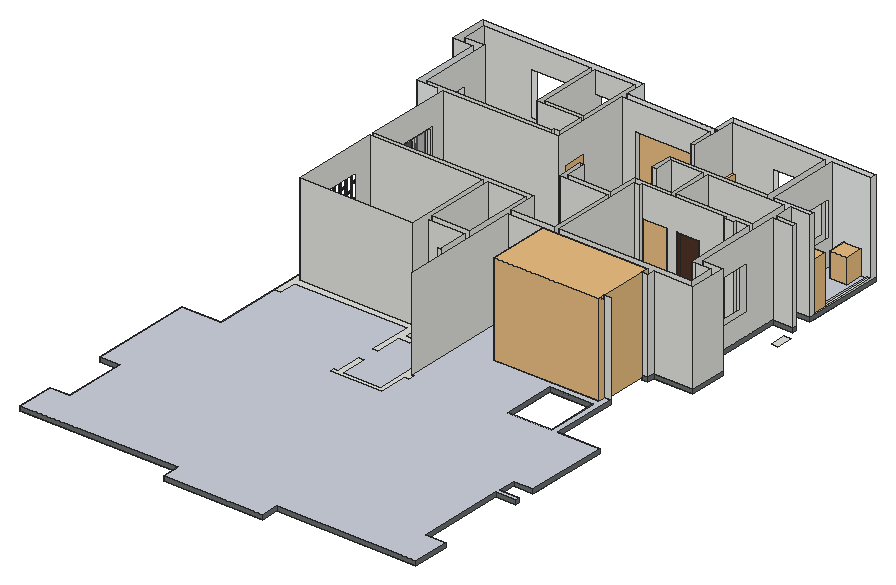
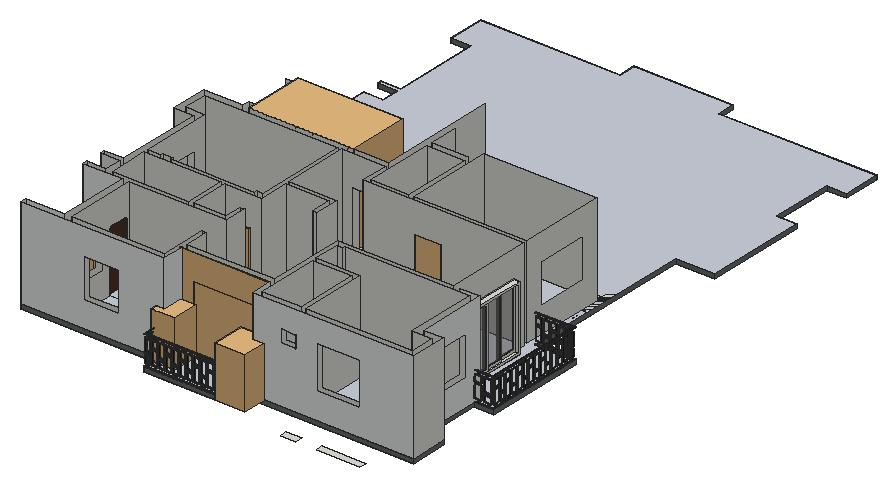
# SketchUp Ruby script. Lengths in inches.
U = 1.inch
M = Sketchup.active_model
def pt(a) = Geom::Point3d.new(a.map { |v| v * U })
def face(e, loops, mat)
  f = e.add_face(loops[0].map { |a| pt(a) })
  loops[1..].each { |l| e.add_face(l.map { |a| pt(a) }).erase! }
  f.material = f.back_material = mat if mat
  f
end
# faces: each face lists its corners as indices into pts; further lists are holes
def faces(e, pts, list, mat = nil) = list.each { |f| face(e, (f[0].is_a?(Array) ? f : [f]).map { |l| l.map { |i| pts[i] } }, mat) }
# xy, xz, yz: faces in a plane at the given z, y or x. An outline is a flat list of corners, or four numbers for a rectangle; further outlines are holes
def ring(l) = l.size == 4 ? [[l[0], l[1]], [l[2], l[1]], [l[2], l[3]], [l[0], l[3]]] : l.each_slice(2).to_a
def flat(e, list, mat, &to3) = list.each { |f| face(e, (f[0].is_a?(Array) ? f : [f]).map { |l| ring(l).map { |u, v| to3.(u, v) } }, mat) }
def xy(e, z, list, mat = nil) = flat(e, list, mat) { |x, y| [x, y, z] }
def xz(e, y, list, mat = nil) = flat(e, list, mat) { |x, z| [x, y, z] }
def yz(e, x, list, mat = nil) = flat(e, list, mat) { |y, z| [x, y, z] }
def lines(e, pts, list) = list.each { |a, b| e.add_line(pt(pts[a]), pt(pts[b])) }
# prism: a flat outline (further loops are holes) pulled along v
def prism(e, loops, v, mat = nil)
  f = face(e, loops, mat); d = Geom::Vector3d.new(v.map { |x| x * U })
  f.pushpull(f.normal.samedirection?(d) ? d.length : -d.length)
end
def box(e, o, s, mat = nil) = prism(e, [[o, [o[0] + s[0], o[1], o[2]], [o[0] + s[0], o[1] + s[1], o[2]], [o[0], o[1] + s[1], o[2]]]], [0, 0, s[2]], mat)
def at(x, y, z, deg = 0) = Geom::Transformation.translation(pt([x, y, z])) * Geom::Transformation.rotation(ORIGIN, Z_AXIS, deg.degrees)
def axes(o, x, y, z) = Geom::Transformation.new([*x, 0, *y, 0, *z, 0, *pt(o).to_a, 1])
def part(name) = M.definitions.add(name)
# library, detail: a bought-in or finely detailed component or shape, given as its bounding box
def library(name, o, s) = part(name).tap { |d| box(d.entities, o, s) }
def detail(e, o, s) = box(e.add_group.entities, o, s)
def put(e, d, t, mat = nil) = e.add_instance(d, t).tap { |i| i.material = mat if mat }
def group(e, t, mat = nil) = e.add_group.tap { |g| g.transformation = t; g.material = mat if mat }.entities
root = M.entities
M.materials.add("1486 AP 8287 DUSK CLOUD").color = [106, 111, 111]
M.materials.add("Polis06_194").color = [79, 50, 36]
M.materials.add("[3P0081_White-City]").color = [235, 238, 238]
M.materials.add("[Color M00]").color = [255, 255, 255]
M.materials.add("[Color M08]").color = [30, 30, 30]
M.materials.add("[Marble Carrara Floor Tile]").color = [204, 208, 219]
M.materials.add("[Translucent Glass Gray]").color = [128, 128, 128]
M.materials["[Translucent Glass Gray]"].alpha = 0.5
c1 = library("Group\#67",[-15,0,-4],[144,84,130])
c2 = part("Flush door")
xy(c2.entities,0,[[0,0,4.72,1.18],[0,34.25,4.72,35.43]],"Polis06_194")
xy(c2.entities,85.26,[[0,1.18,4.72,34.25]],"Polis06_194")
xy(c2.entities,86.61,[[0,0,4.72,35.43]],"Polis06_194")
xz(c2.entities,0,[[0,0,4.72,86.61]],"Polis06_194")
xz(c2.entities,1.18,[[0,0,2.36,85.26],[2.36,0,4.72,85.26]],"Polis06_194")
xz(c2.entities,34.25,[[0,0,4.72,85.26]],"Polis06_194")
xz(c2.entities,35.43,[[0,0,4.72,86.61]],"Polis06_194")
yz(c2.entities,0,[[0,0,1.18,86.61],[34.25,0,35.43,86.61],[1.18,85.26,34.25,86.61]],"Polis06_194")
yz(c2.entities,2.36,[[1.18,0,34.25,0,34.25,85.21,1.18,85.26]],"Polis06_194")
yz(c2.entities,4.72,[[0,0,1.18,86.61],[34.25,0,35.43,86.61],[1.18,85.26,34.25,86.61]],"Polis06_194")
c3 = library("PINTU 6 YA",[0,-0.6875,0],[35.83,8.07,80.71])
c4 = part("구성 요소\#2")
prism(c4.entities,[[[0,0,0],[118.11,0,0],[118.11,0,78.74],[0,0,78.74]],[[116.14,0,76.77],[116.14,0,1.97],[1.97,0,1.97],[1.97,0,76.77]]],[0,7.875,0])
c5 = part("구성 요소\#1")
xy(c5.entities,0,[[[0,0,40.16,74.8],[2.375,2.375,37.78,72.43]]])
xy(c5.entities,1.18,[[2.375,2.375,37.78,72.43]],"[Translucent Glass Gray]")
xy(c5.entities,2.36,[[[0,0,40.16,74.8],[2.375,2.375,37.78,72.43]]])
xz(c5.entities,0,[[0,0,40.16,2.36]],"[Color M00]")
xz(c5.entities,2.375,[[2.375,0,37.78,1.18],[2.375,1.18,37.78,2.36]])
xz(c5.entities,72.43,[[2.375,0,37.78,1.18],[2.375,1.18,37.78,2.36]])
xz(c5.entities,74.8,[[0,0,40.16,2.36]],"[Color M00]")
yz(c5.entities,0,[[0,0,74.8,2.36]])
yz(c5.entities,2.375,[[2.375,0,72.43,1.18],[2.375,1.18,72.43,2.36]])
yz(c5.entities,37.78,[[2.375,0,72.43,1.18],[2.375,1.18,72.43,2.36]])
yz(c5.entities,40.16,[[0,0,74.8,2.36]])
c6 = part("구성 요소\#3")
xy(c6.entities,0,[[0,0,40.16,2.36]],"[Color M00]")
xy(c6.entities,2.375,[[2.375,0,37.78,1.18],[2.375,1.18,37.78,2.36]])
xy(c6.entities,35.83,[[38.48,0,39.47,0.39]])
xy(c6.entities,35.83,[[38.48,1.97,39.47,2.36]],"[Color M00]")
xy(c6.entities,38.98,[[38.48,0,39.47,0.39]])
xy(c6.entities,38.98,[[38.48,1.97,39.47,2.36]],"[Color M00]")
xy(c6.entities,72.43,[[2.375,0,37.78,1.18],[2.375,1.18,37.78,2.36]])
xy(c6.entities,74.8,[[0,0,40.16,2.36]],"[Color M00]")
xz(c6.entities,0,[[[0,0,40.16,74.8],[2.375,2.375,37.78,72.43],[38.48,35.83,39.47,38.98]]])
xz(c6.entities,0.39,[[38.48,35.83,39.47,38.98]])
xz(c6.entities,1.18,[[2.375,2.375,37.78,72.43]],"[Translucent Glass Gray]")
xz(c6.entities,1.97,[[38.48,35.83,39.47,38.98]],"[Color M00]")
xz(c6.entities,2.36,[[[0,0,40.16,74.8],[2.375,2.375,37.78,72.43],[38.48,35.83,39.47,38.98]]])
yz(c6.entities,0,[[0,0,2.36,74.8]])
yz(c6.entities,2.375,[[0,2.375,1.18,72.43],[1.18,2.375,2.36,72.43]])
yz(c6.entities,37.78,[[0,2.375,1.18,72.43],[1.18,2.375,2.36,72.43]])
yz(c6.entities,38.48,[[0,35.83,0.39,38.98]])
yz(c6.entities,38.48,[[1.97,35.83,2.36,38.98]],"[Color M00]")
yz(c6.entities,39.47,[[0,35.83,0.39,38.98]])
yz(c6.entities,39.47,[[1.97,35.83,2.36,38.98]],"[Color M00]")
yz(c6.entities,40.16,[[0,0,2.36,74.8]])
c7 = part("구성 요소\#4")
put(c7.entities,c5,axes([37.78,4.72,0],[1,0,0],[0,0,1],[0,-1,0]))
put(c7.entities,c6,at(75.5625,0,0))
put(c7.entities,c5,axes([0,7.09,0],[1,0,0],[0,0,1],[0,-1,0]))
c8 = part("그룹\#1")
put(c8.entities,c4,axes([0,0,0],[1.04,0,0],[0,1,0],[0,0,1]))
put(c8.entities,c7,axes([1.97,0.39,1.97],[1.02677,0,0],[0,1,0],[0,0,1]))
c9 = part("sliding door")
put(c9.entities,c8,at(0,0,0))
c10 = part("Group\#70")
prism(c10.entities,[[[4.13,0,3.9375],[7.875,0,3.9375],[7.875,0,13.78],[4.13,0,13.78],[4.13,0,15.75],[7.875,0,15.75],[7.875,0,35.43],[4.13,0,35.43],[4.13,0,39.37],[3.74,0,39.37],[3.74,0,35.43],[0,0,35.43],[0,0,15.75],[3.74,0,15.75],[3.74,0,13.78],[0,0,13.78],[0,0,3.9375],[3.74,0,3.9375],[3.74,0,0],[4.13,0,0]],[[0.39,0,16.14],[0.39,0,35.04],[7.48,0,35.04],[7.48,0,16.14]],[[7.48,0,4.33],[0.39,0,4.33],[0.39,0,13.39],[7.48,0,13.39]]],[0,0.39,0],"[Color M08]")
c11 = part("Group\#69")
prism(c11.entities,[[[3.74,0,35.43],[0,0,35.43],[0,0,25.59],[3.74,0,25.59],[3.74,0,23.62],[0,0,23.62],[0,0,3.9375],[3.74,0,3.9375],[3.74,0,0],[4.13,0,0],[4.13,0,3.9375],[7.875,0,3.9375],[7.875,0,23.62],[4.13,0,23.62],[4.13,0,25.59],[7.875,0,25.59],[7.875,0,35.43],[4.13,0,35.43],[4.13,0,39.37],[3.74,0,39.37]],[[7.48,0,23.23],[7.48,0,4.33],[0.39,0,4.33],[0.39,0,23.23]],[[0.39,0,35.04],[7.48,0,35.04],[7.48,0,25.98],[0.39,0,25.98]]],[0,0.39,0],"[Color M08]")
c12 = part("Group\#75")
put(c12.entities,c10,at(0,0,0))
put(c12.entities,c11,at(9.84,0,0))
c13 = part("Group\#76")
put(c13.entities,c10,at(0,0,0))
put(c13.entities,c11,at(9.84,0,0))
c14 = part("Group\#71")
put(c14.entities,c10,at(0,0,0))
put(c14.entities,c11,at(9.84,0,0))
c15 = part("Group\#74")
put(c15.entities,c12,axes([0.79,60.04,0.79],[0,1,0],[1,0,0],[0,0,1]))
put(c15.entities,c12,axes([0.79,40.35,0.79],[0,1,0],[1,0,0],[0,0,1]))
put(c15.entities,c12,axes([0.79,79.72,0.79],[0,1,0],[1,0,0],[0,0,1]))
g1 = group(c15.entities,at(0,0,40.16))
prism(g1,[[[54,-20.92,0],[0,-20.92,0],[0,120.08,0],[27,120.08,0],[27,118.11,0],[1.97,118.11,0],[1.97,-18.98,0],[54,-18.98,0]]],[0,0,0.79],"[Color M08]")
put(c15.entities,c13,axes([0.79,0.98,0.79],[0,1,0],[1,0,0],[0,0,1]))
put(c15.entities,c12,axes([0.79,20.67,0.79],[0,1,0],[1,0,0],[0,0,1]))
put(c15.entities,c12,axes([2.95,118.9,0.79],[1.35733,0,0],[0,1,0],[0,0,1]))
g2 = group(c15.entities,at(0,0,0))
prism(g2,[[[54,-20.92,0],[0,-20.92,0],[0,120.08,0],[27,120.08,0],[27,118.11,0],[1.97,118.11,0],[1.97,-18.98,0],[54,-18.98,0]]],[0,0,0.79],"[Color M08]")
put(c15.entities,c14,axes([0.79,99.41,0.79],[0,1,0],[1,0,0],[0,0,1]))
put(c15.entities,c13,axes([0.79,-18.7,0.79],[0,1,0],[1,0,0],[0,0,1]))
put(c15.entities,c13,axes([22.01,-20.17,0.79],[-1,0,0],[0,1,0],[0,0,1]))
g3 = group(c15.entities,at(43.22,-20.17,0.79))
put(g3,c10,axes([0,0,0],[-1,0,0],[0,1,0],[0,0,1]))
put(g3,c11,axes([-9.84,0,0],[-1,0,0],[0,1,0],[0,0,1]))
put(g3,c11,axes([10.78,0,0],[-1,0,0],[0,1,0],[0,0,1]))
c16 = library("Scara cu plante",[-7.66,-9.41,-0.15],[30.59,22.83,66.38])
c17 = library("Floor panel",[0,13.98,-0.38],[148.62,177.51,16.92])
c18 = library("SLIDING+GLASS+DOOR",[0,-0.75,0],[72,5.75,80])
c19 = library("Group\#241",[0,-0.25,0],[124.5,0.25,126])
c20 = library("Gruppo\#3",[0,0,0],[23.62,24.19,33.46])
c21 = library("Plante 4",[-1.67,-6.5,0],[37.31,31.95,64.42])
c22 = library("cay+chuoi",[26.89,19.66,0.52],[41.96,45.65,69.71])
c23 = part("Group\#81")
g4 = group(c23.entities,at(0,0,0))
prism(g4,[[[24,-19.7,0],[0,-19.7,0],[0,120.08,0],[24,120.08,0],[24,118.11,0],[1.97,118.11,0],[1.97,-17.76,0],[24,-17.76,0]]],[0,0,0.79],"[Color M08]")
put(c23.entities,c14,axes([0.79,40.35,0.79],[0,1,0],[1,0,0],[0,0,1]))
put(c23.entities,c14,at(2.95,118.9,0.79))
put(c23.entities,c14,axes([0.79,79.72,0.79],[0,1,0],[1,0,0],[0,0,1]))
put(c23.entities,c14,axes([0.79,60.04,0.79],[0,1,0],[1,0,0],[0,0,1]))
put(c23.entities,c14,axes([0.79,99.41,0.79],[0,1,0],[1,0,0],[0,0,1]))
put(c23.entities,c14,axes([0.79,0.98,0.79],[0,1,0],[1,0,0],[0,0,1]))
g5 = group(c23.entities,at(0,0,40.16))
prism(g5,[[[24,-19.7,0],[0,-19.7,0],[0,120.08,0],[24,120.08,0],[24,118.11,0],[1.97,118.11,0],[1.97,-17.76,0],[24,-17.76,0]]],[0,0,0.79],"[Color M08]")
put(c23.entities,c14,axes([0.79,20.67,0.79],[0,1,0],[1,0,0],[0,0,1]))
put(c23.entities,c14,axes([0.79,-18.7,0.79],[0,1,0],[1,0,0],[0,0,1]))
put(c23.entities,c14,axes([2.95,-18.49,0.79],[1,0,0],[0,-1,0],[0,0,1]))
xy(root,228,[[382.75,774.97,404.25,783.97],[649.5,1017.47,658.5,1038.97],[218,1143.97,278,1152.97],[306,1143.97,327.5,1152.97]])
xy(root,258,[[[144,357.97,366,357.97,366,387.97,490.5,387.97,490.5,357.97,688.5,357.97,688.5,408.97,661.5,408.97,661.5,529,688.5,529,688.5,535,661.5,535,661.5,558.97,688.5,558.97,688.5,564.97,631.5,564.97,631.5,663.97,688.5,663.97,688.5,672.97,631.5,672.97,631.5,763.97,622.5,763.97,622.5,753.97,553.5,753.97,553.5,738.97,562.5,738.97,562.5,744.97,622.5,744.97,622.5,672.97,562.5,672.97,562.5,678.97,553.5,678.97,553.5,672.97,430.5,672.97,430.5,837.97,622.5,837.97,622.5,827.97,631.5,827.97,631.5,837.97,685.5,837.97,685.5,888.97,658.5,888.97,658.5,1009,685.5,1009,685.5,1015,658.5,1015,658.5,1038.97,649.5,1038.97,649.5,984.97,544.5,984.97,544.5,1038.97,685.5,1038.97,685.5,1044.97,631.5,1044.97,631.5,1143.97,685.5,1143.97,685.5,1152.97,487.5,1152.97,487.5,1122.97,366,1122.97,366,1152.97,144,1152.97,144,1101.97,171,1101.97,171,1005.97,198,1005.97,198,504.97,171,504.97,171,408.97,144,408.97],[366,396.97,366,504.97,207,504.97,207,624.97,427.5,624.97,427.5,663.97,487.5,663.97,487.5,572.47,421.5,572.47,421.5,537.97,427.5,537.97,427.5,566.47,487.5,566.47,487.5,537.97,493.5,537.97,493.5,663.97,622.5,663.97,622.5,564.97,541.5,564.97,541.5,504.97,490.5,504.97,490.5,396.97],[427.5,846.97,427.5,885.97,207,885.97,207,1005.97,366,1005.97,366,1113.97,487.5,1113.97,487.5,1080.97,493.5,1080.97,493.5,1143.97,622.5,1143.97,622.5,1044.97,487.5,1044.97,487.5,1014.97,493.5,1014.97,493.5,1038.97,538.5,1038.97,538.5,984.97,487.5,984.97,487.5,944.47,427.5,944.47,427.5,972.97,421.5,972.97,421.5,938.47,487.5,938.47,487.5,846.97],[496.5,366.97,496.5,495.97,504.5,495.97,504.5,498.97,617.5,498.97,617.5,495.97,631.5,495.97,631.5,498.97,652.5,498.97,652.5,399.97,679.5,399.97,679.5,366.97],[493.5,846.97,493.5,975.97,501.5,975.97,501.5,978.97,617.5,978.97,617.5,975.97,631.5,975.97,631.5,978.97,649.5,978.97,649.5,879.97,676.5,879.97,676.5,846.97],[207,630.97,207,750.97,372,750.97,372,774.97,421.5,774.97,421.5,735.97,372,735.97,372,750.97,363,750.97,363,630.97],[180,1011.97,180,1110.97,153,1110.97,153,1143.97,300,1143.97,300,1050.97,360,1050.97,360,1014.97,352,1014.97,352,1011.97],[153,366.97,153,399.97,180,399.97,180,498.97,352,498.97,352,495.97,360,495.97,360,459.97,300,459.97,300,366.97],[207,759.97,363,879.97],[547.5,504.97,652.5,558.97],[369,783.97,421.5,879.97],[369,630.97,421.5,726.97],[306,366.97,360,453.97],[306,1056.97,360,1143.97]]])
xy(root,264,[[357,624.97,357,630.97,363,630.97,363,666.97,369,666.97,369,630.97,421.5,630.97,421.5,726.97,404.25,726.97,404.25,735.97,421.5,735.97,421.5,774.97,404.25,774.97,404.25,783.97,421.5,783.97,421.5,879.97,369,879.97,369,843.97,363,843.97,363,879.97,357,879.97,357,885.97,427.5,885.97,427.5,846.97,433.5,846.97,433.5,837.97,430.5,837.97,430.5,672.97,433.5,672.97,433.5,663.97,427.5,663.97,427.5,624.97],[363,690.97,363,750.97,207,750.97,207,726.97,198,726.97,198,785.97,207,785.97,207,759.97,363,759.97,363,819.97,369,819.97,369,783.97,384.75,783.97,384.75,774.97,372,774.97,372,735.97,384.75,735.97,384.75,726.97,369,726.97,369,690.97],[384.75,774.97,402.25,778.97],[402.25,774.97,404.25,783.97],[384.75,778.97,402.25,779.97],
  [384.75,779.97,402.25,783.97],[198,785.97,202,853.97],[202,785.97,203,853.97],[203,785.97,207,853.97],[622.5,827.97,622.5,837.97,472.5,837.97,472.5,846.97,487.5,846.97,487.5,938.47,421.5,938.47,421.5,972.97,427.5,972.97,427.5,944.47,487.5,944.47,487.5,984.97,504,984.97,504,978.97,501.5,978.97,501.5,975.97,493.5,975.97,493.5,846.97,676.5,846.97,676.5,879.97,649.5,879.97,649.5,897.97,658.5,897.97,658.5,888.97,685.5,888.97,685.5,837.97,631.5,837.97,631.5,827.97],
  [198,853.97,207,855.97],[198,855.97,198,903.97,207,903.97,207,885.97,321,885.97,321,879.97,207,879.97,207,855.97],[649.5,897.97,658.5,899.97],[649.5,899.97,653.5,961.97],[653.5,899.97,654.5,961.97],
  [654.5,899.97,658.5,961.97],[649.5,961.97,649.5,978.97,631.5,978.97,631.5,975.97,617.5,975.97,617.5,978.97,580.5,978.97,580.5,984.97,649.5,984.97,649.5,1019.47,658.5,1019.47,658.5,1015,685.5,1015,685.5,1009,658.5,1009,658.5,961.97],[536,978.97,536,984.97,538.5,984.97,538.5,1038.97,493.5,1038.97,493.5,1014.97,487.5,1014.97,487.5,1044.97,622.5,1044.97,622.5,1047.97,631.5,1047.97,631.5,1044.97,685.5,1044.97,685.5,1038.97,544.5,1038.97,544.5,984.97,550.5,984.97,550.5,978.97],[649.5,1019.47,653.5,1036.97],[653.5,1019.47,654.5,1036.97],
  [654.5,1019.47,658.5,1036.97],[171,1029.97,180,1031.97],[171,1031.97,175,1075.97],[175,1031.97,176,1075.97],[176,1031.97,180,1075.97],
  [649.5,1036.97,658.5,1038.97],[679.5,1044.97,679.5,1143.97,631.5,1143.97,631.5,1077.97,622.5,1077.97,622.5,1143.97,598.5,1143.97,598.5,1152.97,685.5,1152.97,685.5,1044.97],[300,1050.97,300,1143.97,278,1143.97,278,1152.97,306,1152.97,306,1056.97,309,1056.97,309,1050.97],[171,1075.97,180,1077.97],[171,1077.97,171,1101.97,144,1101.97,144,1152.97,220,1152.97,220,1143.97,153,1143.97,153,1110.97,180,1110.97,180,1077.97],
  [487.5,1080.97,487.5,1113.97,470.25,1113.97,470.25,1122.97,487.5,1122.97,487.5,1152.97,552.5,1152.97,552.5,1143.97,493.5,1143.97,493.5,1086.97,513.5,1086.97,513.5,1080.97],[220,1143.97,276,1147.97],[276,1143.97,278,1152.97],[306,1143.97,308,1152.97],[308,1143.97,325.5,1147.97],
  [325.5,1143.97,327.5,1152.97],[552.5,1143.97,596.5,1147.97],[596.5,1143.97,598.5,1152.97],[220,1147.97,276,1148.97],[308,1147.97,325.5,1148.97],
  [552.5,1147.97,596.5,1148.97],[220,1148.97,276,1152.97],[308,1148.97,325.5,1152.97],[552.5,1148.97,596.5,1152.97]])
xz(root,759.97,[[207,264,363,390]])
xz(root,763.97,[[622.5,264,631.5,390]])
xz(root,774.97,[[[372,264,421.5,390],[382.75,342,404.25,360]]])
xz(root,783.97,[[[369,264,421.5,390],[382.75,342,404.25,360]]])
xz(root,819.97,[[363,264,369,348]])
xz(root,827.97,[[622.5,264,631.5,390]])
xz(root,837.97,[[430.5,264,433.5,264,433.5,348,472.5,348,472.5,264,622.5,264,622.5,390,430.5,390],[631.5,264,685.5,390]])
xz(root,843.97,[[363,264,369,348]])
xz(root,846.97,[[427.5,264,427.5,390,487.5,390,487.5,264,472.5,264,472.5,348,433.5,348,433.5,264],[493.5,264,676.5,390]])
xz(root,879.97,[[207,264,321,264,321,348,357,348,357,264,363,264,363,390,207,390],[369,264,421.5,390],[649.5,264,654.5,390],[654.5,264,676.5,390]])
xz(root,885.97,[[207,264,207,390,427.5,390,427.5,264,357,264,357,348,321,348,321,264]])
xz(root,888.97,[[658.5,264,685.5,390]])
xz(root,903.97,[[198,264,207,354]])
xz(root,938.47,[[421.5,264,487.5,390]])
xz(root,944.47,[[427.5,264,487.5,390]])
xz(root,972.97,[[421.5,264,427.5,390]])
xz(root,975.97,[[493.5,264,501.5,390],[617.5,264,631.5,390]])
xz(root,978.97,[[501.5,264,504,264,504,348,536,348,536,264,550.5,264,550.5,348,580.5,348,580.5,264,617.5,264,617.5,390,501.5,390],[631.5,264,649.5,390]])
xz(root,984.97,[[487.5,264,487.5,390,538.5,390,538.5,264,536,264,536,348,504,348,504,264],[544.5,264,544.5,390,649.5,390,649.5,264,580.5,264,580.5,348,550.5,348,550.5,264]])
xz(root,987.97,[[198,264,207,354]])
xz(root,1005.97,[[207,264,366,390]])
xz(root,1005.97,[[171,264,198,390]],"[3P0081_White-City]")
xz(root,1009,[[658.5,264,685.5,390]])
xz(root,1011.97,[[180,264,352,390]])
xz(root,1014.97,[[352,264,360,390],[487.5,264,493.5,390]])
xz(root,1015,[[658.5,264,685.5,390]])
xz(root,1017.47,[[360,264,366,348]])
xz(root,1038.97,[[493.5,264,538.5,390],[544.5,264,649.5,264,649.5,342,658.5,342,658.5,264,685.5,264,685.5,390,658.5,390,658.5,360,649.5,360,649.5,390,544.5,390]])
xz(root,1044.97,[[487.5,264,622.5,390]])
xz(root,1044.97,[[631.5,264,631.5,390,685.5,390,685.5,266,679.5,266,679.5,264]],"[3P0081_White-City]")
xz(root,1047.47,[[360,264,366,348]])
xz(root,1047.97,[[622.5,264,631.5,348]])
xz(root,1050.97,[[300,264,309,264,309,348,333,348,333,264,360,264,360,390,300,390]])
xz(root,1056.97,[[306,264,306,390,360,390,360,264,333,264,333,348,309,348,309,264]])
xz(root,1077.97,[[622.5,264,631.5,348]])
xz(root,1080.97,[[487.5,264,513.5,264,513.5,300,493.5,300,493.5,390,487.5,390]])
xz(root,1086.97,[[493.5,264,513.5,300]])
xz(root,1101.97,[[144,264,171,390]])
xz(root,1110.97,[[153,264,180,390]])
xz(root,1113.97,[[366,264,386.25,264,386.25,354,470.25,354,470.25,264,487.5,264,487.5,390,366,390]])
xz(root,1122.97,[[366,264,366,390,487.5,390,487.5,264,470.25,264,470.25,354,386.25,354,386.25,264]],"[3P0081_White-City]")
xz(root,1143.97,[[[153,264,300,390],[218,300,278,360]],[306,264,360,264,360,390,306,390,306,360,327.5,360,327.5,342,306,342],[[493.5,264,622.5,390],[550.5,300,598.5,354]]])
xz(root,1143.97,[[631.5,264,679.5,264,679.5,266,685.5,266,685.5,390,631.5,390]],"[3P0081_White-City]")
xz(root,1152.97,[[[144,264,366,390],[218,300,278,360],[306,342,327.5,360]],[[487.5,264,685.5,390],[550.5,300,598.5,354]]],"[3P0081_White-City]")
yz(root,144,[[1101.97,264,1152.97,390]])
yz(root,153,[[1110.97,264,1143.97,390]])
yz(root,171,[[[1005.97,264,1101.97,390],[1029.97,300,1077.97,354]]],"[3P0081_White-City]")
yz(root,180,[[[1011.97,264,1110.97,390],[1029.97,300,1077.97,354]]])
yz(root,207,[[[759.97,264,879.97,390],[783.97,300,855.97,354]],[885.97,264,903.97,264,903.97,354,987.97,354,987.97,264,1005.97,264,1005.97,390,885.97,390]])
yz(root,300,[[1050.97,264,1143.97,390]])
yz(root,306,[[1056.97,264,1143.97,264,1143.97,342,1152.97,342,1152.97,360,1143.97,360,1143.97,390,1056.97,390]])
yz(root,309,[[1050.97,264,1056.97,348]])
yz(root,321,[[879.97,264,885.97,348]])
yz(root,333,[[1050.97,264,1056.97,348]])
yz(root,352,[[1011.97,264,1014.97,390]])
yz(root,357,[[879.97,264,885.97,348]])
yz(root,360,[[1014.97,264,1014.97,390,1050.97,390,1050.97,264,1047.47,264,1047.47,348,1017.47,348,1017.47,264],[1056.97,264,1143.97,390]])
yz(root,363,[[759.97,264,759.97,390,879.97,390,879.97,264,843.97,264,843.97,348,819.97,348,819.97,264]])
yz(root,366,[[1005.97,264,1017.47,264,1017.47,348,1047.47,348,1047.47,264,1113.97,264,1113.97,390,1005.97,390]])
yz(root,366,[[1122.97,264,1152.97,390]],"[3P0081_White-City]")
yz(root,369,[[783.97,264,819.97,264,819.97,348,843.97,348,843.97,264,879.97,264,879.97,390,783.97,390]])
yz(root,386.25,[[1113.97,264,1122.97,354]])
yz(root,421.5,[[735.97,264,774.97,390],[783.97,264,879.97,390],[938.47,264,972.97,390]])
yz(root,427.5,[[846.97,264,885.97,390],[944.47,264,972.97,390]])
yz(root,430.5,[[672.97,264,837.97,390]])
yz(root,433.5,[[837.97,264,846.97,348]])
yz(root,470.25,[[1113.97,264,1122.97,354]])
yz(root,472.5,[[837.97,264,846.97,348]])
yz(root,487.5,[[846.97,264,938.47,390],[944.47,264,984.97,390],[1014.97,264,1044.97,390],[1080.97,264,1113.97,390]])
yz(root,487.5,[[1122.97,264,1152.97,390]],"[3P0081_White-City]")
yz(root,493.5,[[846.97,264,975.97,390],[1014.97,264,1038.97,390],[1086.97,264,1143.97,264,1143.97,390,1080.97,390,1080.97,300,1086.97,300]])
yz(root,501.5,[[975.97,264,978.97,390]])
yz(root,504,[[978.97,264,984.97,348]])
yz(root,513.5,[[1080.97,264,1086.97,300]])
yz(root,536,[[978.97,264,984.97,348]])
yz(root,538.5,[[984.97,264,1038.97,390]])
yz(root,544.5,[[984.97,264,1038.97,390]])
yz(root,550.5,[[978.97,264,984.97,348]])
yz(root,580.5,[[978.97,264,984.97,348]])
yz(root,617.5,[[975.97,264,978.97,390]])
yz(root,622.5,[[753.97,264,763.97,390],[827.97,264,837.97,390],[[1044.97,264,1044.97,390,1143.97,390,1143.97,264,1077.97,264,1077.97,348,1047.97,348,1047.97,264],[1089.97,300,1137.97,348]]])
yz(root,631.5,[[827.97,264,837.97,390],[975.97,264,978.97,390],[[1044.97,264,1047.97,264,1047.97,348,1077.97,348,1077.97,264,1143.97,264,1143.97,390,1044.97,390],[1089.97,300,1137.97,348]]])
yz(root,649.5,[[[879.97,264,978.97,390],[897.97,294,963.97,354]],[984.97,264,984.97,390,1038.97,390,1038.97,360,1017.47,360,1017.47,342,1038.97,342,1038.97,264]])
yz(root,658.5,[[[888.97,264,1009,390],[897.97,294,963.97,354]],[1015,264,1038.97,264,1038.97,342,1017.47,342,1017.47,360,1038.97,360,1038.97,390,1015,390]])
yz(root,676.5,[[846.97,264,879.97,390]])
yz(root,679.5,[[1044.97,264,1143.97,266]])
yz(root,685.5,[[837.97,264,888.97,390],[1009,264,1015,390],[1038.97,264,1152.97,264,1152.97,390,1143.97,390,1143.97,266,1044.97,266,1044.97,390,1038.97,390]])
p = [[511.5,1086.97,264],[511.5,1119.97,264],[487.5,964.47,264],[427.5,964.47,264],[474.5,938.47,264],[474.5,846.97,264],
  [598.5,1077.97,264],[598.5,1119.97,264],[654.5,846.97,264],[654.5,879.97,264],[175,1143.97,264],[175,1110.97,264],
  [538.5,1018.97,264],[493.5,1018.97,264],[388.25,1113.97,264],[388.25,1122.97,264],[202.5,932.97,264],[202.5,931.97,264],
  [203.5,932.97,264],[622.5,1077.97,264],[470.25,1113.97,264],[468.25,1113.97,264],[200.5,958.97,264],[201.5,958.97,264],
  [468.25,1119.97,264],[427.25,1119.97,264],[386.25,1122.97,264],[468.25,1122.97,264],[446.25,1117.97,264],[446.25,1118.97,264],
  [406.25,1117.97,264],[363,817.97,264],[341,817.97,264],[406.25,1118.97,264],[200.5,985.97,264],[207,905.97,264],
  [203.5,905.97,264],[487.5,1080.97,264],[487.5,1044.97,264],[421.5,885.97,264],[421.5,938.47,264],[207,987.97,264],
  [207,985.97,264],[300,1050.97,264],[300,1011.97,264],[198,985.97,264],[201.5,960.47,264],[427.25,1118.97,264],
  [201.5,931.97,264],[198,903.97,264],[198,905.97,264],[202.5,960.47,264],[306,1050.97,264],[306,1011.97,264],
  [493.5,1014.97,264],[493.5,984.97,264],[487.5,1014.97,264],[487.5,984.97,264],[341,759.97,264],[493.5,1080.97,264],
  [493.5,1044.97,264],[427.5,885.97,264],[427.5,938.47,264],[421.5,774.97,264],[396.75,755.47,264],[372,774.97,264],
  [207,903.97,264],[201.5,985.97,264],[468.25,1118.97,264],[202.5,905.97,264],[386.25,1113.97,264],[470.25,1122.97,264],
  [198,987.97,264]]
lines(root,p,[[0,1],[2,3],[4,5],[6,7],[8,9],[10,11],[12,13],[14,15],[16,17],[18,16],[6,19],[20,21],
  [22,23],[24,25],[26,15],[27,24],[28,29],[30,28],[31,32],[33,30],[34,22],[35,36],[37,38],[39,40],
  [41,42],[36,18],[43,44],[45,34],[46,23],[25,47],[47,29],[48,17],[49,50],[51,46],[52,53],[54,55],
  [56,57],[32,58],[59,60],[61,62],[63,64],[65,64],[15,27],[21,14],[16,51],[35,66],[34,67],[50,45],
  [24,68],[68,21],[23,48],[47,33],[17,69],[46,67],[29,68],[69,50],[14,70],[42,35],[36,69],[7,1],
  [27,71],[45,72],[67,42]])
g6 = group(root,at(144,357.97,270),"1486 AP 8287 DUSK CLOUD")
xy(g6,-12,[[[216,-24,216,0,0,0,0,51,27,51,27,136.5,0,136.5,0,277.5,54,277.5,54,517.5,0,517.5,0,658.5,27,658.5,27,744,0,744,0,795,216,795,216,819,352.5,819,352.5,795,541.5,795,541.5,786,487.5,786,487.5,687,541.5,687,541.5,681,514.5,681,514.5,657.03,541.5,657.03,541.5,651.03,514.5,651.03,514.5,531,541.5,531,541.5,480,487.5,480,487.5,470,478.5,470,478.5,480,340.5,480,340.5,396,478.5,396,478.5,406,487.5,406,487.5,315,544.5,315,544.5,306,487.5,306,487.5,207,544.5,207,544.5,201,517.5,201,517.5,177.03,544.5,177.03,544.5,171.03,517.5,171.03,517.5,51,544.5,51,544.5,0,352.5,0,352.5,-24],[222,-18,346.5,30],[225,766.57,340.5,816],[418.5,315,478.5,387]],[[487.5,207,544.5,306],[490.5,210,541.5,303]],[[487.5,687,541.5,786],[490.5,690,538.5,783]]])
xy(g6,-9,[[222,-18,346.5,30],[490.5,210,541.5,303],[490.5,690,538.5,783],[225,766.57,340.5,816]])
xy(g6,-6,[[[216,-24,352.5,-24,352.5,0,544.5,0,544.5,51,517.5,51,517.5,171.03,544.5,171.03,544.5,177.03,517.5,177.03,517.5,201,544.5,201,544.5,315,487.5,315,487.5,406,478.5,406,478.5,396,340.5,396,340.5,480,478.5,480,478.5,470,487.5,470,487.5,480,541.5,480,541.5,531,514.5,531,514.5,651.03,541.5,651.03,541.5,657.03,514.5,657.03,514.5,681,541.5,681,541.5,795,352.5,795,352.5,819,216,819,216,795,0,795,0,744,27,744,27,658.5,0,658.5,0,517.5,54,517.5,54,277.5,0,277.5,0,136.5,27,136.5,27,51,0,51,0,0,216,0],[418.5,315,478.5,387]]],"[Marble Carrara Floor Tile]")
xz(g6,-24,[[216,-12,352.5,-6]])
xz(g6,-18,[[222,-12,346.5,-9]])
xz(g6,0,[[0,-12,216,-6],[352.5,-12,544.5,-6]])
xz(g6,30,[[222,-12,346.5,-9]])
xz(g6,51,[[0,-12,27,-6],[517.5,-12,544.5,-6]])
xz(g6,136.5,[[0,-12,27,-6]])
xz(g6,171.03,[[517.5,-12,544.5,-6]])
xz(g6,177.03,[[517.5,-12,544.5,-6]])
xz(g6,201,[[517.5,-12,544.5,-6]])
xz(g6,210,[[490.5,-12,541.5,-9]])
xz(g6,277.5,[[0,-12,54,-6]])
xz(g6,303,[[490.5,-12,541.5,-9]])
xz(g6,315,[[418.5,-12,478.5,-6],[487.5,-12,544.5,-6]])
xz(g6,387,[[418.5,-12,478.5,-6]])
xz(g6,396,[[340.5,-12,478.5,-6]])
xz(g6,406,[[478.5,-12,487.5,-6]])
xz(g6,470,[[478.5,-12,487.5,-6]])
xz(g6,480,[[340.5,-12,478.5,-6],[487.5,-12,541.5,-6]])
xz(g6,517.5,[[0,-12,54,-6]])
xz(g6,531,[[514.5,-12,541.5,-6]])
xz(g6,651.03,[[514.5,-12,541.5,-6]])
xz(g6,657.03,[[514.5,-12,541.5,-6]])
xz(g6,658.5,[[0,-12,27,-6]])
xz(g6,681,[[514.5,-12,541.5,-6]])
xz(g6,690,[[490.5,-12,538.5,-9]])
xz(g6,744,[[0,-12,27,-6]])
xz(g6,766.57,[[225,-12,340.5,-9]])
xz(g6,783,[[490.5,-12,538.5,-9]])
xz(g6,795,[[0,-12,216,-6],[352.5,-12,541.5,-6]])
xz(g6,816,[[225,-12,340.5,-9]])
xz(g6,819,[[216,-12,352.5,-6]])
yz(g6,0,[[0,-12,51,-6],[136.5,-12,277.5,-6],[517.5,-12,658.5,-6],[744,-12,795,-6]])
yz(g6,27,[[51,-12,136.5,-6],[658.5,-12,744,-6]])
yz(g6,54,[[277.5,-12,517.5,-6]])
yz(g6,216,[[-24,-12,0,-6],[795,-12,819,-6]])
yz(g6,222,[[-18,-12,30,-9]])
yz(g6,225,[[766.57,-12,816,-9]])
yz(g6,340.5,[[396,-12,480,-6],[766.57,-12,816,-9]])
yz(g6,346.5,[[-18,-12,30,-9]])
yz(g6,352.5,[[-24,-12,0,-6],[795,-12,819,-6]])
yz(g6,418.5,[[315,-12,387,-6]])
yz(g6,478.5,[[315,-12,387,-6],[396,-12,406,-6],[470,-12,480,-6]])
yz(g6,487.5,[[315,-12,406,-6],[470,-12,480,-6]])
yz(g6,490.5,[[210,-12,303,-9],[690,-12,783,-9]])
yz(g6,514.5,[[531,-12,651.03,-6],[657.03,-12,681,-6]])
yz(g6,517.5,[[51,-12,171.03,-6],[177.03,-12,201,-6]])
yz(g6,538.5,[[690,-12,783,-9]])
yz(g6,541.5,[[210,-12,303,-9],[480,-12,531,-6],[651.03,-12,657.03,-6],[681,-12,795,-6]])
yz(g6,544.5,[[0,-12,51,-6],[171.03,-12,177.03,-6],[201,-12,315,-6]])
p = [[343.5,765,-12],[222,765,-12]]
lines(g6,p,[[0,1]])
put(root,c1,at(493.5,753.97,264))
put(root,c2,axes([367.72,819.97,264],[-1,0,0],[0,0.67733,0],[0,0,0.96982]))
put(root,c3,axes([321,885.29,264],[1.00475,0,0],[0,-1,0],[0,0,1.04078]))
put(root,c9,axes([198,903.97,264],[0,0.68385,0],[1,0,0],[0,0,1.143]))
put(root,c15,axes([144,896.4,264],[1,0,0],[0,1,0],[0,0,0.97692]))
put(root,c2,axes([580.5,984.39,264],[0,-1,0],[-0.84667,0,0],[0,0,0.96982]))
put(root,c3,axes([536,979.66,264],[-0.89311,0,0],[0,1,0],[0,0,1.04078]))
put(root,c3,axes([365.3125,1047.96,264],[0.01802,-0.8369,0],[-0.99977,-0.02153,0],[0,0,1.04078]))
put(root,c2,axes([333,1052.25,264],[0,1,0],[-0.67733,0,0],[0,0,0.96982]))
put(root,c16,axes([660.01,1058.41,264],[1,0,0],[0,-1,0],[0,0,1]))
put(root,c2,axes([627.22,1077.97,264],[-1,0,0],[0,-0.84667,0],[0,0,0.96982]))
put(root,c17,axes([634.5,1040.65,258.32],[0.32297,0,0],[0,0.52389,0],[0,0,0.27]))
put(root,c18,axes([386.25,1122.97,264],[1.16667,0,0],[0,-1,0],[0,0,1.125]))
put(root,c19,axes([366,1122.97,264],[1,0,0],[0,-1,0],[0,0,1]))
put(root,c20,at(647.91,1119.78,264))
put(root,c21,at(491.29,1126.79,264,90))
put(root,c17,axes([493.59,1174.04,256.54],[0,-0.33306,0],[-0.65064,0,0],[0,0,0.27]))
put(root,c22,at(323.18,1120.82,263.22))
put(root,c23,axes([477.26,1176.97,264],[0,-1,0],[-0.97654,0,0],[0,0,1]))
